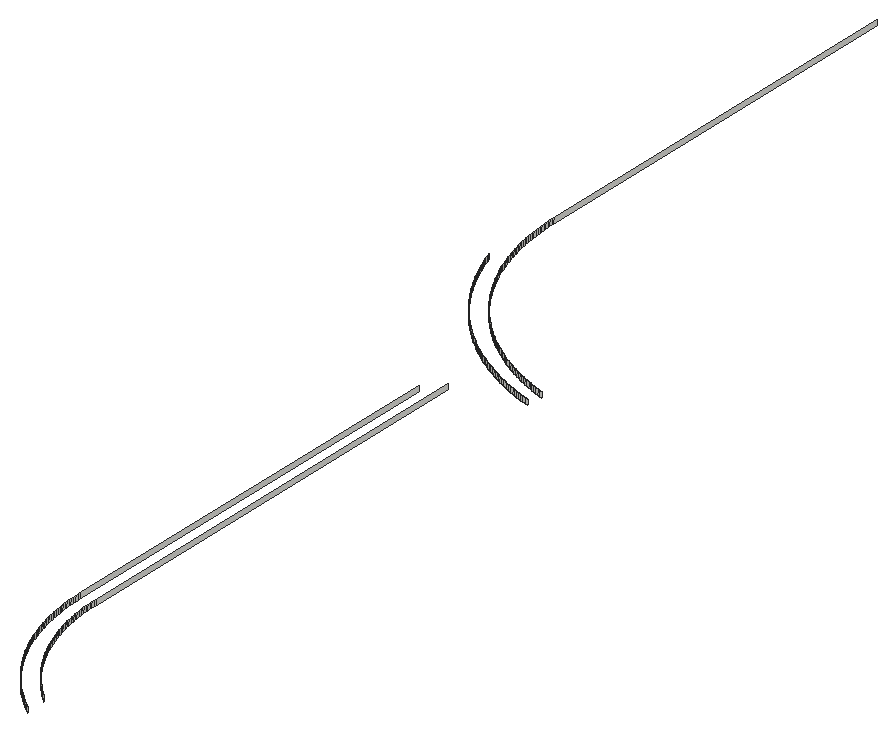
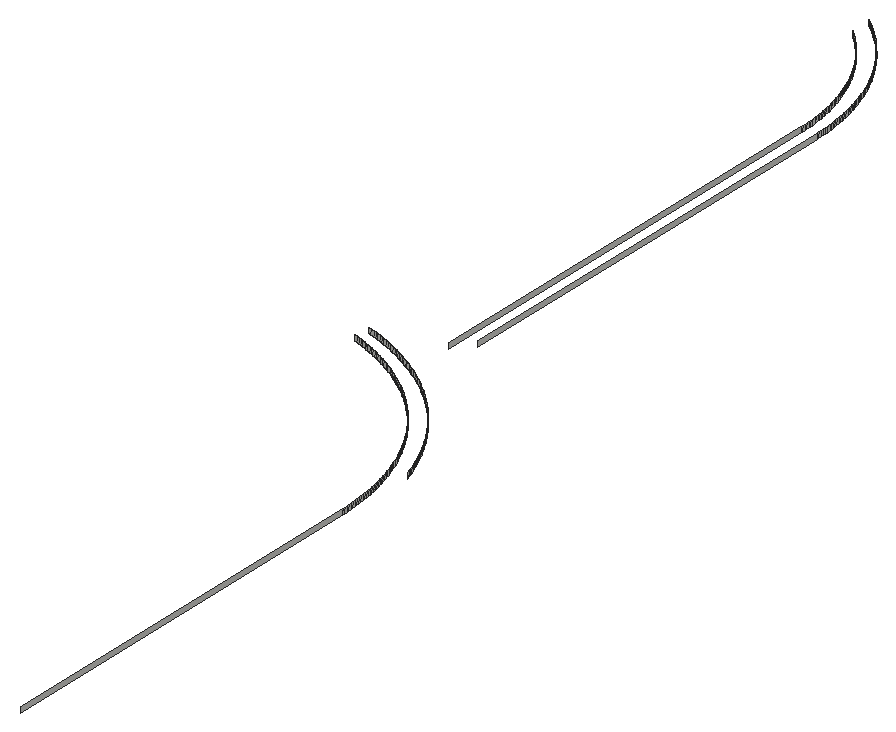
# SketchUp Ruby script. Lengths in inches.
U = 1.inch
M = Sketchup.active_model
def pt(a) = Geom::Point3d.new(a.map { |v| v * U })
def face(e, loops, mat)
  f = e.add_face(loops[0].map { |a| pt(a) })
  loops[1..].each { |l| e.add_face(l.map { |a| pt(a) }).erase! }
  f.material = f.back_material = mat if mat
  f
end
# faces: each face lists its corners as indices into pts; further lists are holes
def faces(e, pts, list, mat = nil) = list.each { |f| face(e, (f[0].is_a?(Array) ? f : [f]).map { |l| l.map { |i| pts[i] } }, mat) }
# xy, xz, yz: faces in a plane at the given z, y or x. An outline is a flat list of corners, or four numbers for a rectangle; further outlines are holes
def ring(l) = l.size == 4 ? [[l[0], l[1]], [l[2], l[1]], [l[2], l[3]], [l[0], l[3]]] : l.each_slice(2).to_a
def flat(e, list, mat, &to3) = list.each { |f| face(e, (f[0].is_a?(Array) ? f : [f]).map { |l| ring(l).map { |u, v| to3.(u, v) } }, mat) }
def xy(e, z, list, mat = nil) = flat(e, list, mat) { |x, y| [x, y, z] }
def xz(e, y, list, mat = nil) = flat(e, list, mat) { |x, z| [x, y, z] }
def yz(e, x, list, mat = nil) = flat(e, list, mat) { |y, z| [x, y, z] }
def lines(e, pts, list) = list.each { |a, b| e.add_line(pt(pts[a]), pt(pts[b])) }
# prism: a flat outline (further loops are holes) pulled along v
def prism(e, loops, v, mat = nil)
  f = face(e, loops, mat); d = Geom::Vector3d.new(v.map { |x| x * U })
  f.pushpull(f.normal.samedirection?(d) ? d.length : -d.length)
end
def box(e, o, s, mat = nil) = prism(e, [[o, [o[0] + s[0], o[1], o[2]], [o[0] + s[0], o[1] + s[1], o[2]], [o[0], o[1] + s[1], o[2]]]], [0, 0, s[2]], mat)
def at(x, y, z, deg = 0) = Geom::Transformation.translation(pt([x, y, z])) * Geom::Transformation.rotation(ORIGIN, Z_AXIS, deg.degrees)
def axes(o, x, y, z) = Geom::Transformation.new([*x, 0, *y, 0, *z, 0, *pt(o).to_a, 1])
def part(name) = M.definitions.add(name)
# library, detail: a bought-in or finely detailed component or shape, given as its bounding box
def library(name, o, s) = part(name).tap { |d| box(d.entities, o, s) }
def detail(e, o, s) = box(e.add_group.entities, o, s)
def put(e, d, t, mat = nil) = e.add_instance(d, t).tap { |i| i.material = mat if mat }
def group(e, t, mat = nil) = e.add_group.tap { |g| g.transformation = t; g.material = mat if mat }.entities
root = M.entities
yz(root,130,[[209.73,116,209.95,116.5],[209.95,116,209.99,116.5],[209.99,116,248,116.5]])
yz(root,130.01,[[209.2,116,209.47,116.5]])
yz(root,138,[[143.74,116,144,116.5],[144,116,184,116.5]])
yz(root,139.5,[[143.76,116,144,116.5],[144,116,185.5,116.5]])
yz(root,139.51,[[143.27,116,143.52,116.5]])
p = [[145.62,128.29,116],[145.41,128.46,116],[145.41,128.46,116.5],[145.62,128.29,116.5],[145.21,128.625,116],[145.21,128.625,116.5],
  [145.01,128.79,116],[145.01,128.79,116.5],[144.8125,128.96,116],[144.8125,128.96,116.5],[144.62,129.14,116],[144.62,129.14,116.5],
  [144.42,129.3125,116],[144.42,129.3125,116.5],[144.23,129.49,116],[144.23,129.49,116.5],[144.04,129.67,116],[144.04,129.67,116.5],
  [143.86,129.86,116],[143.86,129.86,116.5],[143.67,130.04,116],[143.67,130.04,116.5],[143.49,130.23,116],[143.49,130.23,116.5],
  [143.3125,130.42,116],[143.3125,130.42,116.5],[145.44,130.42,116],[145.62,130.25,116],[145.62,130.25,116.5],[145.44,130.42,116.5],
  [143.14,130.62,116],[143.14,130.62,116.5],[145.27,130.58,116],[145.27,130.58,116.5],[142.96,130.8125,116],[142.96,130.8125,116.5],
  [145.09,130.75,116],[145.09,130.75,116.5],[144.92,130.92,116],[144.92,130.92,116.5],[142.79,131.01,116],[142.79,131.01,116.5],
  [144.75,131.09,116],[144.75,131.09,116.5],[142.625,131.21,116],[142.625,131.21,116.5],[144.58,131.27,116],[144.58,131.27,116.5],
  [142.46,131.41,116],[142.46,131.41,116.5],[144.42,131.44,116],[144.42,131.44,116.5],[142.29,131.62,116],[142.29,131.62,116.5],
  [144.25,131.62,116],[144.25,131.62,116.5],[142.13,131.82,116],[142.13,131.82,116.5],[144.09,131.8,116],[144.09,131.8,116.5],
  [141.97,132.03,116],[141.97,132.03,116.5],[143.93,131.99,116],[143.93,131.99,116.5],[141.82,132.24,116],[141.82,132.24,116.5],
  [143.78,132.17,116],[143.78,132.17,116.5],[141.67,132.46,116],[141.67,132.46,116.5],[143.62,132.36,116],[143.62,132.36,116.5],
  [143.47,132.55,116],[143.47,132.55,116.5],[141.52,132.67,116],[141.52,132.67,116.5],[143.32,132.74,116],[143.32,132.74,116.5],
  [141.37,132.89,116],[141.37,132.89,116.5],[143.18,132.93,116],[143.18,132.93,116.5],[141.23,133.11,116],[141.23,133.11,116.5],
  [143.03,133.125,116],[143.03,133.125,116.5],[141.09,133.33,116],[141.09,133.33,116.5],[142.89,133.32,116],[142.89,133.32,116.5],
  [140.95,133.55,116],[140.95,133.55,116.5],[142.75,133.52,116],[142.75,133.52,116.5],[142.62,133.72,116],[142.62,133.72,116.5],
  [140.8125,133.77,116],[140.8125,133.77,116.5],[142.48,133.92,116],[142.48,133.92,116.5],[140.68,134,116],[140.68,134,116.5],
  [142.35,134.13,116],[142.35,134.13,116.5],[140.55,134.23,116],[140.55,134.23,116.5],[142.23,134.33,116],[142.23,134.33,116.5],
  [140.42,134.46,116],[140.42,134.46,116.5],[142.1,134.54,116],[142.1,134.54,116.5],[140.3,134.6875,116],[140.3,134.6875,116.5],
  [141.98,134.75,116],[141.98,134.75,116.5],[140.18,134.92,116],[140.18,134.92,116.5],[141.86,134.96,116],[141.86,134.96,116.5],
  [140.0625,135.15,116],[140.0625,135.15,116.5],[141.74,135.17,116],[141.74,135.17,116.5],[139.95,135.39,116],[139.95,135.39,116.5],
  [141.63,135.39,116],[141.63,135.39,116.5],[139.84,135.625,116],[139.84,135.625,116.5],[141.52,135.6,116],[141.52,135.6,116.5],
  [139.73,135.87,116],[139.73,135.87,116.5],[141.41,135.82,116],[141.41,135.82,116.5],[141.3,136.04,116],[141.3,136.04,116.5],
  [139.625,136.11,116],[139.625,136.11,116.5],[141.2,136.25,116],[141.2,136.25,116.5],[139.52,136.35,116],[139.52,136.35,116.5],
  [139.42,136.59,116],[139.42,136.59,116.5],[141.1,136.48,116],[141.1,136.48,116.5],[141,136.7,116],[141,136.7,116.5],
  [139.33,136.83,116],[139.33,136.83,116.5],[140.91,136.92,116],[140.91,136.92,116.5],[139.24,137.08,116],[139.24,137.08,116.5],
  [140.82,137.14,116],[140.82,137.14,116.5],[139.15,137.32,116],[139.15,137.32,116.5],[140.73,137.37,116],[140.73,137.37,116.5],
  [139.0625,137.57,116],[139.0625,137.57,116.5],[140.64,137.6,116],[140.64,137.6,116.5],[138.98,137.82,116],[138.98,137.82,116.5],
  [140.5625,137.82,116],[140.5625,137.82,116.5],[138.9,138.07,116],[138.9,138.07,116.5],[140.48,138.05,116],[140.48,138.05,116.5],
  [138.82,138.32,116],[138.82,138.32,116.5],[140.41,138.28,116],[140.41,138.28,116.5],[138.75,138.57,116],[138.75,138.57,116.5],
  [140.33,138.51,116],[140.33,138.51,116.5],[140.26,138.75,116],[140.26,138.75,116.5],[138.68,138.82,116],[138.68,138.82,116.5],
  [140.19,138.98,116],[140.19,138.98,116.5],[138.62,139.08,116],[138.62,139.08,116.5],[140.13,139.21,116],[140.13,139.21,116.5],
  [138.55,139.33,116],[138.55,139.33,116.5],[140.07,139.45,116],[140.07,139.45,116.5],[138.49,139.59,116],[138.49,139.59,116.5],
  [140.01,139.68,116],[140.01,139.68,116.5],[138.4375,139.84,116],[138.4375,139.84,116.5],[139.96,139.92,116],[139.96,139.92,116.5],
  [138.38,140.1,116],[138.38,140.1,116.5],[139.9,140.15,116],[139.9,140.15,116.5],[138.33,140.36,116],[138.33,140.36,116.5],
  [139.86,140.39,116],[139.86,140.39,116.5],[138.29,140.61,116],[138.29,140.61,116.5],[139.81,140.63,116],[139.81,140.63,116.5],
  [138.25,140.87,116],[138.25,140.87,116.5],[139.77,140.87,116],[139.77,140.87,116.5],[138.21,141.13,116],[138.21,141.13,116.5],
  [139.73,141.11,116],[139.73,141.11,116.5],[138.17,141.39,116],[138.17,141.39,116.5],[139.69,141.35,116],[139.69,141.35,116.5],
  [139.66,141.59,116],[139.66,141.59,116.5],[138.14,141.65,116],[138.14,141.65,116.5],[138.11,141.91,116],[138.11,141.91,116.5],
  [139.63,141.83,116],[139.63,141.83,116.5],[139.6,142.07,116],[139.6,142.07,116.5],[138.08,142.17,116],[138.08,142.17,116.5],
  [139.58,142.31,116],[139.58,142.31,116.5],[138.0625,142.43,116],[138.0625,142.43,116.5],[139.56,142.55,116],[139.56,142.55,116.5],
  [138.04,142.69,116],[138.04,142.69,116.5],[139.54,142.79,116],[139.54,142.79,116.5],[138.03,142.95,116],[138.03,142.95,116.5],
  [139.53,143.03,116],[139.53,143.03,116.5],[138.02,143.21,116],[138.02,143.21,116.5],[139.51,143.27,116],[139.51,143.27,116.5],
  [138.01,143.48,116],[138.01,143.48,116.5],[138,143.74,116],[138,143.74,116.5],[139.5,143.76,116],[139.51,143.52,116],
  [139.51,143.52,116.5],[139.5,143.76,116.5],[145.55,187.4,116],[145.28,187.48,116],[145.28,187.48,116.5],[145.55,187.4,116.5],
  [145.01,187.5625,116],[145.01,187.5625,116.5],[144.74,187.65,116],[144.74,187.65,116.5],[144.47,187.74,116],[144.2,187.83,116],
  [144.2,187.83,116.5],[144.47,187.74,116.5],[143.93,187.93,116],[143.93,187.93,116.5],[143.67,188.03,116],[143.67,188.03,116.5],
  [143.4,188.13,116],[143.4,188.13,116.5],[143.14,188.23,116],[143.14,188.23,116.5],[142.875,188.34,116],[142.875,188.34,116.5],
  [142.61,188.46,116],[142.61,188.46,116.5],[142.36,188.57,116],[142.36,188.57,116.5],[142.1,188.6875,116],[142.1,188.6875,116.5],
  [141.84,188.81,116],[141.84,188.81,116.5],[141.58,188.93,116],[141.58,188.93,116.5],[141.33,189.0625,116],[141.33,189.0625,116.5],
  [145.45,189,116],[145.71,188.92,116],[145.71,188.92,116.5],[145.45,189,116.5],[145.2,189.08,116],[145.2,189.08,116.5],
  [141.08,189.19,116],[141.08,189.19,116.5],[144.95,189.16,116],[144.95,189.16,116.5],[140.83,189.33,116],[140.83,189.33,116.5],
  [144.45,189.34,116],[144.7,189.25,116],[144.7,189.25,116.5],[144.45,189.34,116.5],[140.58,189.46,116],[140.58,189.46,116.5],
  [144.2,189.43,116],[144.2,189.43,116.5],[143.95,189.53,116],[143.95,189.53,116.5],[140.33,189.6,116],[140.33,189.6,116.5],
  [143.7,189.625,116],[143.7,189.625,116.5],[140.09,189.74,116],[140.09,189.74,116.5],[143.46,189.73,116],[143.46,189.73,116.5],
  [139.84,189.89,116],[139.84,189.89,116.5],[143.21,189.83,116],[143.21,189.83,116.5],[142.97,189.9375,116],[142.97,189.9375,116.5],
  [139.6,190.04,116],[139.6,190.04,116.5],[142.73,190.05,116],[142.73,190.05,116.5],[139.36,190.1875,116],[139.36,190.1875,116.5],
  [142.49,190.16,116],[142.49,190.16,116.5],[139.12,190.34,116],[139.12,190.34,116.5],[142.25,190.28,116],[142.25,190.28,116.5],
  [138.89,190.5,116],[138.89,190.5,116.5],[142.01,190.4,116],[142.01,190.4,116.5],[141.78,190.52,116],[141.78,190.52,116.5],
  [138.65,190.66,116],[138.65,190.66,116.5],[141.54,190.64,116],[141.54,190.64,116.5],[141.31,190.77,116],[141.31,190.77,116.5],
  [138.42,190.82,116],[138.42,190.82,116.5],[138.1875,190.99,116],[138.1875,190.99,116.5],[141.08,190.9,116],[141.08,190.9,116.5],
  [140.85,191.04,116],[140.85,191.04,116.5],[137.96,191.16,116],[137.96,191.16,116.5],[140.62,191.17,116],[140.62,191.17,116.5],
  [137.73,191.33,116],[137.73,191.33,116.5],[140.39,191.3125,116],[140.39,191.3125,116.5],[137.51,191.5,116],[137.51,191.5,116.5],
  [140.17,191.45,116],[140.17,191.45,116.5],[137.28,191.68,116],[137.28,191.68,116.5],[139.94,191.6,116],[139.94,191.6,116.5],
  [139.72,191.74,116],[139.72,191.74,116.5],[137.0625,191.86,116],[137.0625,191.86,116.5],[139.5,191.89,116],[139.5,191.89,116.5],
  [136.85,192.04,116],[136.85,192.04,116.5],[139.28,192.05,116],[139.28,192.05,116.5],[136.63,192.22,116],[136.63,192.22,116.5],
  [139.07,192.2,116],[139.07,192.2,116.5],[136.42,192.41,116],[136.42,192.41,116.5],[138.85,192.36,116],[138.85,192.36,116.5],
  [136.21,192.6,116],[136.21,192.6,116.5],[138.64,192.52,116],[138.64,192.52,116.5],[138.43,192.68,116],[138.43,192.68,116.5],
  [136,192.79,116],[136,192.79,116.5],[138.22,192.85,116],[138.22,192.85,116.5],[135.79,192.99,116],[135.79,192.99,116.5],
  [138.02,193.01,116],[138.02,193.01,116.5],[135.58,193.18,116],[135.58,193.18,116.5],[137.8125,193.18,116],[137.8125,193.18,116.5],
  [135.38,193.38,116],[135.38,193.38,116.5],[137.61,193.36,116],[137.61,193.36,116.5],[135.18,193.58,116],[135.18,193.58,116.5],
  [137.41,193.53,116],[137.41,193.53,116.5],[137.21,193.71,116],[137.21,193.71,116.5],[134.99,193.79,116],[134.99,193.79,116.5],
  [137.02,193.89,116],[137.02,193.89,116.5],[134.79,194,116],[134.79,194,116.5],[136.82,194.07,116],[136.82,194.07,116.5],
  [134.6,194.21,116],[134.6,194.21,116.5],[136.63,194.26,116],[136.63,194.26,116.5],[134.41,194.42,116],[134.41,194.42,116.5],
  [136.44,194.44,116],[136.44,194.44,116.5],[134.22,194.63,116],[134.22,194.63,116.5],[136.26,194.63,116],[136.26,194.63,116.5],
  [134.04,194.85,116],[134.04,194.85,116.5],[136.07,194.82,116],[136.07,194.82,116.5],[133.86,195.0625,116],[133.86,195.0625,116.5],
  [135.89,195.02,116],[135.89,195.02,116.5],[135.71,195.21,116],[135.71,195.21,116.5],[133.68,195.28,116],[133.68,195.28,116.5],
  [135.53,195.41,116],[135.53,195.41,116.5],[133.5,195.51,116],[133.5,195.51,116.5],[135.36,195.61,116],[135.36,195.61,116.5],
  [133.33,195.73,116],[133.33,195.73,116.5],[135.18,195.8125,116],[135.18,195.8125,116.5],[133.16,195.96,116],[133.16,195.96,116.5],
  [135.01,196.02,116],[135.01,196.02,116.5],[132.99,196.1875,116],[132.99,196.1875,116.5],[134.85,196.22,116],[134.85,196.22,116.5],
  [132.82,196.42,116],[132.82,196.42,116.5],[134.68,196.43,116],[134.68,196.43,116.5],[132.66,196.65,116],[132.66,196.65,116.5],
  [134.52,196.64,116],[134.52,196.64,116.5],[134.36,196.85,116],[134.36,196.85,116.5],[132.5,196.89,116],[132.5,196.89,116.5],
  [132.34,197.12,116],[132.34,197.12,116.5],[134.2,197.07,116],[134.2,197.07,116.5],[132.1875,197.36,116],[132.1875,197.36,116.5],
  [134.05,197.28,116],[134.05,197.28,116.5],[133.89,197.5,116],[133.89,197.5,116.5],[132.04,197.6,116],[132.04,197.6,116.5],
  [133.74,197.72,116],[133.74,197.72,116.5],[131.89,197.84,116],[131.89,197.84,116.5],[133.6,197.94,116],[133.6,197.94,116.5],
  [131.74,198.09,116],[131.74,198.09,116.5],[133.45,198.17,116],[133.45,198.17,116.5],[131.6,198.33,116],[131.6,198.33,116.5],
  [133.3125,198.39,116],[133.3125,198.39,116.5],[131.46,198.58,116],[131.46,198.58,116.5],[133.17,198.62,116],[133.17,198.62,116.5],
  [131.33,198.83,116],[131.33,198.83,116.5],[133.04,198.85,116],[133.04,198.85,116.5],[131.19,199.08,116],[131.19,199.08,116.5],
  [132.9,199.08,116],[132.9,199.08,116.5],[131.0625,199.33,116],[131.0625,199.33,116.5],[132.77,199.31,116],[132.77,199.31,116.5],
  [130.93,199.58,116],[130.93,199.58,116.5],[132.64,199.54,116],[132.64,199.54,116.5],[132.52,199.78,116],[132.52,199.78,116.5],
  [130.81,199.84,116],[130.81,199.84,116.5],[130.6875,200.1,116],[130.6875,200.1,116.5],[132.4,200.01,116],[132.4,200.01,116.5],
  [132.28,200.25,116],[132.28,200.25,116.5],[130.57,200.36,116],[130.57,200.36,116.5],[132.16,200.49,116],[132.16,200.49,116.5],
  [130.46,200.61,116],[130.46,200.61,116.5],[132.05,200.73,116],[132.05,200.73,116.5],[130.34,200.875,116],[130.34,200.875,116.5],
  [131.9375,200.97,116],[131.9375,200.97,116.5],[130.23,201.14,116],[130.23,201.14,116.5],[131.83,201.21,116],[131.83,201.21,116.5],
  [130.13,201.4,116],[130.13,201.4,116.5],[131.73,201.46,116],[131.73,201.46,116.5],[130.03,201.67,116],[130.03,201.67,116.5],
  [131.625,201.7,116],[131.625,201.7,116.5],[129.93,201.93,116],[129.93,201.93,116.5],[131.53,201.95,116],[131.53,201.95,116.5],
  [129.83,202.2,116],[129.83,202.2,116.5],[131.43,202.2,116],[131.43,202.2,116.5],[129.74,202.47,116],[129.74,202.47,116.5],
  [131.34,202.45,116],[131.34,202.45,116.5],[131.25,202.7,116],[131.25,202.7,116.5],[129.65,202.74,116],[129.65,202.74,116.5],
  [131.16,202.95,116],[131.16,202.95,116.5],[131.08,203.2,116],[131.08,203.2,116.5],[131,203.45,116],[131,203.45,116.5],
  [130.92,203.71,116],[130.92,203.71,116.5],[130.84,203.96,116],[130.84,203.96,116.5],[130.77,204.22,116],[130.77,204.22,116.5],
  [130.7,204.48,116],[130.7,204.48,116.5],[130.64,204.74,116],[130.64,204.74,116.5],[130.58,204.99,116],[130.58,204.99,116.5],
  [130.52,205.25,116],[130.52,205.25,116.5],[130.46,205.51,116],[130.46,205.51,116.5],[130.41,205.77,116],[130.41,205.77,116.5],
  [130.36,206.03,116],[130.36,206.03,116.5],[130.3125,206.3,116],[130.3125,206.3,116.5],[130.27,206.56,116],[130.27,206.56,116.5],
  [130.23,206.82,116],[130.23,206.82,116.5],[130.19,207.08,116],[130.19,207.08,116.5],[130.16,207.35,116],[130.16,207.35,116.5],
  [130.13,207.61,116],[130.13,207.61,116.5],[130.1,207.875,116],[130.1,207.875,116.5],[130.08,208.14,116],[130.08,208.14,116.5],
  [130.06,208.41,116],[130.06,208.41,116.5],[130.04,208.67,116],[130.04,208.67,116.5],[130.03,208.9375,116],[130.03,208.9375,116.5],
  [130.01,209.2,116],[130.01,209.2,116.5],[130,209.73,116],[130.01,209.47,116],[130.01,209.47,116.5],[130,209.73,116.5]]
faces(root,p,[[0,1,2,3],[1,4,5,2],[4,6,7,5],[6,8,9,7],[8,10,11,9],[10,12,13,11],[12,14,15,13],[14,16,17,15],
  [16,18,19,17],[18,20,21,19],[20,22,23,21],[22,24,25,23],[26,27,28,29],[24,30,31,25],[32,26,29,33],[30,34,35,31],
  [36,32,33,37],[38,36,37,39],[34,40,41,35],[42,38,39,43],[40,44,45,41],[46,42,43,47],[44,48,49,45],[50,46,47,51],
  [48,52,53,49],[54,50,51,55],[52,56,57,53],[58,54,55,59],[56,60,61,57],[62,58,59,63],[60,64,65,61],[66,62,63,67],
  [64,68,69,65],[70,66,67,71],[72,70,71,73],[68,74,75,69],[76,72,73,77],[74,78,79,75],[80,76,77,81],[78,82,83,79],
  [84,80,81,85],[82,86,87,83],[88,84,85,89],[86,90,91,87],[92,88,89,93],[94,92,93,95],[90,96,97,91],[98,94,95,99],
  [96,100,101,97],[102,98,99,103],[100,104,105,101],[106,102,103,107],[104,108,109,105],[110,106,107,111],[108,112,113,109],[114,110,111,115],
  [112,116,117,113],[118,114,115,119],[116,120,121,117],[122,118,119,123],[120,124,125,121],[126,122,123,127],[124,128,129,125],[130,126,127,131],
  [128,132,133,129],[134,130,131,135],[136,134,135,137],[132,138,139,133],[140,136,137,141],[138,142,143,139],[142,144,145,143],[146,140,141,147],
  [148,146,147,149],[144,150,151,145],[152,148,149,153],[150,154,155,151],[156,152,153,157],[154,158,159,155],[160,156,157,161],[158,162,163,159],
  [164,160,161,165],[162,166,167,163],[168,164,165,169],[166,170,171,167],[172,168,169,173],[170,174,175,171],[176,172,173,177],[174,178,179,175],
  [180,176,177,181],[182,180,181,183],[178,184,185,179],[186,182,183,187],[184,188,189,185],[190,186,187,191],[188,192,193,189],[194,190,191,195],
  [192,196,197,193],[198,194,195,199],[196,200,201,197],[202,198,199,203],[200,204,205,201],[206,202,203,207],[204,208,209,205],[210,206,207,211],
  [208,212,213,209],[214,210,211,215],[212,216,217,213],[218,214,215,219],[216,220,221,217],[222,218,219,223],[220,224,225,221],[226,222,223,227],
  [228,226,227,229],[224,230,231,225],[230,232,233,231],[234,228,229,235],[236,234,235,237],[232,238,239,233],[240,236,237,241],[238,242,243,239],
  [244,240,241,245],[242,246,247,243],[248,244,245,249],[246,250,251,247],[252,248,249,253],[250,254,255,251],[256,252,253,257],[254,258,259,255],
  [258,260,261,259],[262,263,264,265],[266,267,268,269],[267,270,271,268],[270,272,273,271],[274,275,276,277],[272,274,277,273],[275,278,279,276],
  [278,280,281,279],[280,282,283,281],[282,284,285,283],[284,286,287,285],[286,288,289,287],[288,290,291,289],[290,292,293,291],[292,294,295,293],
  [294,296,297,295],[296,298,299,297],[300,301,302,303],[304,300,303,305],[298,306,307,299],[308,304,305,309],[306,310,311,307],[312,313,314,315],
  [313,308,309,314],[310,316,317,311],[318,312,315,319],[320,318,319,321],[316,322,323,317],[324,320,321,325],[322,326,327,323],[328,324,325,329],
  [326,330,331,327],[332,328,329,333],[334,332,333,335],[330,336,337,331],[338,334,335,339],[336,340,341,337],[342,338,339,343],[340,344,345,341],
  [346,342,343,347],[344,348,349,345],[350,346,347,351],[352,350,351,353],[348,354,355,349],[356,352,353,357],[358,356,357,359],[354,360,361,355],
  [360,362,363,361],[364,358,359,365],[366,364,365,367],[362,368,369,363],[370,366,367,371],[368,372,373,369],[374,370,371,375],[372,376,377,373],
  [378,374,375,379],[376,380,381,377],[382,378,379,383],[384,382,383,385],[380,386,387,381],[388,384,385,389],[386,390,391,387],[392,388,389,393],
  [390,394,395,391],[396,392,393,397],[394,398,399,395],[400,396,397,401],[398,402,403,399],[404,400,401,405],[406,404,405,407],[402,408,409,403],
  [410,406,407,411],[408,412,413,409],[414,410,411,415],[412,416,417,413],[418,414,415,419],[416,420,421,417],[422,418,419,423],[420,424,425,421],
  [426,422,423,427],[428,426,427,429],[424,430,431,425],[432,428,429,433],[430,434,435,431],[436,432,433,437],[434,438,439,435],[440,436,437,441],
  [438,442,443,439],[444,440,441,445],[442,446,447,443],[448,444,445,449],[446,450,451,447],[452,448,449,453],[450,454,455,451],[456,452,453,457],
  [458,456,457,459],[454,460,461,455],[462,458,459,463],[460,464,465,461],[466,462,463,467],[464,468,469,465],[470,466,467,471],[468,472,473,469],
  [474,470,471,475],[472,476,477,473],[478,474,475,479],[476,480,481,477],[482,478,479,483],[480,484,485,481],[486,482,483,487],[488,486,487,489],
  [484,490,491,485],[490,492,493,491],[494,488,489,495],[492,496,497,493],[498,494,495,499],[500,498,499,501],[496,502,503,497],[504,500,501,505],
  [502,506,507,503],[508,504,505,509],[506,510,511,507],[512,508,509,513],[510,514,515,511],[516,512,513,517],[514,518,519,515],[520,516,517,521],
  [518,522,523,519],[524,520,521,525],[522,526,527,523],[528,524,525,529],[526,530,531,527],[532,528,529,533],[530,534,535,531],[536,532,533,537],
  [538,536,537,539],[534,540,541,535],[540,542,543,541],[544,538,539,545],[546,544,545,547],[542,548,549,543],[550,546,547,551],[548,552,553,549],
  [554,550,551,555],[552,556,557,553],[558,554,555,559],[556,560,561,557],[562,558,559,563],[560,564,565,561],[566,562,563,567],[564,568,569,565],
  [570,566,567,571],[568,572,573,569],[574,570,571,575],[572,576,577,573],[578,574,575,579],[576,580,581,577],[582,578,579,583],[584,582,583,585],
  [580,586,587,581],[588,584,585,589],[590,588,589,591],[592,590,591,593],[594,592,593,595],[596,594,595,597],[598,596,597,599],[600,598,599,601],
  [602,600,601,603],[604,602,603,605],[606,604,605,607],[608,606,607,609],[610,608,609,611],[612,610,611,613],[614,612,613,615],[616,614,615,617],
  [618,616,617,619],[620,618,619,621],[622,620,621,623],[624,622,623,625],[626,624,625,627],[628,626,627,629],[630,628,629,631],[632,630,631,633],
  [634,632,633,635],[636,634,635,637],[638,639,640,641]])
